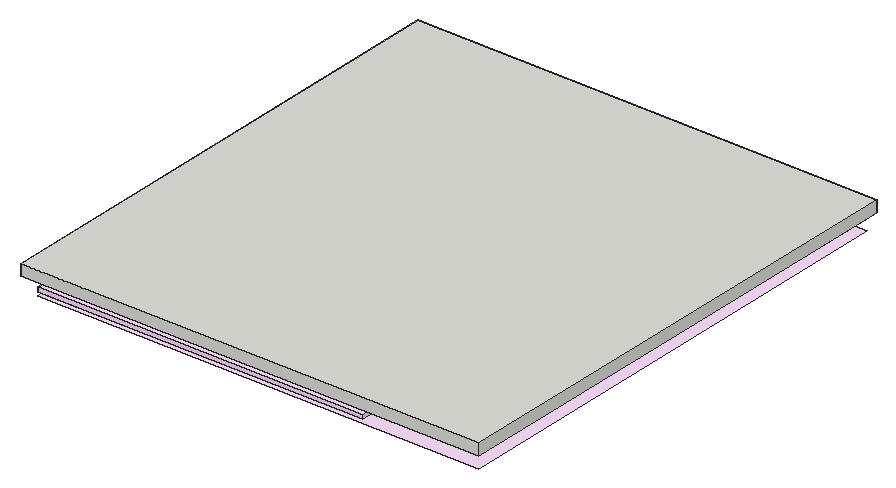
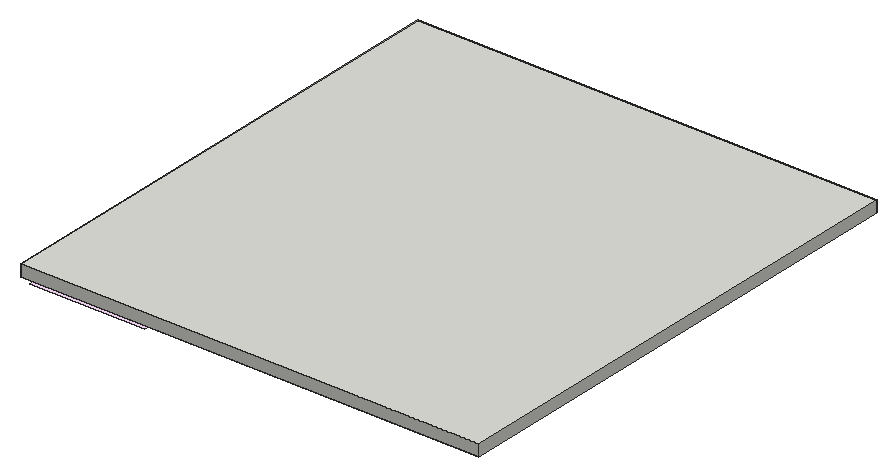
# SketchUp Ruby script. Lengths in inches.
U = 1.inch
M = Sketchup.active_model
def pt(a) = Geom::Point3d.new(a.map { |v| v * U })
def face(e, loops, mat)
  f = e.add_face(loops[0].map { |a| pt(a) })
  loops[1..].each { |l| e.add_face(l.map { |a| pt(a) }).erase! }
  f.material = f.back_material = mat if mat
  f
end
# faces: each face lists its corners as indices into pts; further lists are holes
def faces(e, pts, list, mat = nil) = list.each { |f| face(e, (f[0].is_a?(Array) ? f : [f]).map { |l| l.map { |i| pts[i] } }, mat) }
# xy, xz, yz: faces in a plane at the given z, y or x. An outline is a flat list of corners, or four numbers for a rectangle; further outlines are holes
def ring(l) = l.size == 4 ? [[l[0], l[1]], [l[2], l[1]], [l[2], l[3]], [l[0], l[3]]] : l.each_slice(2).to_a
def flat(e, list, mat, &to3) = list.each { |f| face(e, (f[0].is_a?(Array) ? f : [f]).map { |l| ring(l).map { |u, v| to3.(u, v) } }, mat) }
def xy(e, z, list, mat = nil) = flat(e, list, mat) { |x, y| [x, y, z] }
def xz(e, y, list, mat = nil) = flat(e, list, mat) { |x, z| [x, y, z] }
def yz(e, x, list, mat = nil) = flat(e, list, mat) { |y, z| [x, y, z] }
def lines(e, pts, list) = list.each { |a, b| e.add_line(pt(pts[a]), pt(pts[b])) }
# prism: a flat outline (further loops are holes) pulled along v
def prism(e, loops, v, mat = nil)
  f = face(e, loops, mat); d = Geom::Vector3d.new(v.map { |x| x * U })
  f.pushpull(f.normal.samedirection?(d) ? d.length : -d.length)
end
def box(e, o, s, mat = nil) = prism(e, [[o, [o[0] + s[0], o[1], o[2]], [o[0] + s[0], o[1] + s[1], o[2]], [o[0], o[1] + s[1], o[2]]]], [0, 0, s[2]], mat)
def at(x, y, z, deg = 0) = Geom::Transformation.translation(pt([x, y, z])) * Geom::Transformation.rotation(ORIGIN, Z_AXIS, deg.degrees)
def axes(o, x, y, z) = Geom::Transformation.new([*x, 0, *y, 0, *z, 0, *pt(o).to_a, 1])
def part(name) = M.definitions.add(name)
# library, detail: a bought-in or finely detailed component or shape, given as its bounding box
def library(name, o, s) = part(name).tap { |d| box(d.entities, o, s) }
def detail(e, o, s) = box(e.add_group.entities, o, s)
def put(e, d, t, mat = nil) = e.add_instance(d, t).tap { |i| i.material = mat if mat }
def group(e, t, mat = nil) = e.add_group.tap { |g| g.transformation = t; g.material = mat if mat }.entities
root = M.entities
M.materials.add("[0118_Thistle]").color = [255, 225, 255]
M.materials.add("[Color M00]").color = [255, 255, 255]
xy(root,116.0625,[[[48.73,154.34,48.21,154.4,47.73,154.6,47.32,154.92,47,155.34,46.8,155.82,46.73,156.34,46.8,156.85,47,157.34,47.32,157.75,47.73,158.07,48.21,158.27,48.73,158.34,49.25,158.27,49.73,158.07,50.15,157.75,50.46,157.34,50.66,156.85,50.73,156.34,50.66,155.82,50.46,155.34,50.15,154.92,49.73,154.6,49.25,154.4],[48.73,154.84,49.12,154.89,49.48,155.04,49.79,155.28,50.03,155.59,50.18,155.95,50.23,156.34,50.18,156.72,50.03,157.09,49.79,157.4,49.48,157.64,49.12,157.79,48.73,157.84,48.34,157.79,47.98,157.64,47.67,157.4,47.43,157.09,47.28,156.72,47.23,156.34,47.28,155.95,47.43,155.59,47.67,155.28,47.98,155.04,48.34,154.89]]],"[Color M00]")
xy(root,116.125,[[[32.11,108.44,31.6,108.51,31.11,108.71,30.7,109.03,30.38,109.44,30.18,109.93,30.11,110.44,30.18,110.96,30.38,111.44,30.7,111.86,31.11,112.18,31.6,112.375,32.11,112.44,32.63,112.375,33.11,112.18,33.53,111.86,33.85,111.44,34.05,110.96,34.11,110.44,34.05,109.93,33.85,109.44,33.53,109.03,33.11,108.71,32.63,108.51],[32.11,108.94,32.5,108.99,32.86,109.14,33.17,109.38,33.41,109.69,33.5625,110.06,33.61,110.44,33.5625,110.83,33.41,111.19,33.17,111.5,32.86,111.74,32.5,111.89,32.11,111.94,31.73,111.89,31.36,111.74,31.05,111.5,30.81,111.19,30.66,110.83,30.61,110.44,30.66,110.06,30.81,109.69,31.05,109.38,31.36,109.14,31.73,108.99]],[[178.2,146.39,177.6875,146.46,177.2,146.66,176.79,146.97,176.47,147.39,176.27,147.87,176.2,148.39,176.27,148.91,176.47,149.39,176.79,149.8,177.2,150.12,177.6875,150.32,178.2,150.39,178.72,150.32,179.2,150.12,179.62,149.8,179.9375,149.39,180.14,148.91,180.2,148.39,180.14,147.87,179.9375,147.39,179.62,146.97,179.2,146.66,178.72,146.46],[178.2,146.89,178.59,146.94,178.95,147.09,179.26,147.33,179.5,147.64,179.65,148,179.7,148.39,179.65,148.78,179.5,149.14,179.26,149.45,178.95,149.6875,178.59,149.84,178.2,149.89,177.82,149.84,177.45,149.6875,177.14,149.45,176.91,149.14,176.76,148.78,176.7,148.39,176.76,148,176.91,147.64,177.14,147.33,177.45,147.09,177.82,146.94]],[[126.7,154.34,126.1875,154.4,125.7,154.6,125.29,154.92,124.97,155.34,124.77,155.82,124.7,156.34,124.77,156.85,124.97,157.34,125.29,157.75,125.7,158.07,126.1875,158.27,126.7,158.34,127.22,158.27,127.7,158.07,128.12,157.75,128.44,157.34,128.64,156.85,128.7,156.34,128.64,155.82,128.44,155.34,128.12,154.92,127.7,154.6,127.22,154.4],[126.7,154.82,127.1,154.87,127.46,155.02,127.78,155.26,128.02,155.58,128.17,155.94,128.22,156.34,128.17,156.73,128.02,157.09,127.78,157.41,127.46,157.65,127.1,157.8,126.7,157.85,126.3125,157.8,125.94,157.65,125.63,157.41,125.39,157.09,125.24,156.73,125.1875,156.34,125.24,155.94,125.39,155.58,125.63,155.26,125.94,155.02,126.3125,154.87]]],"[Color M00]")
xy(root,116.1875,[[[160.13,91.36,159.62,91.43,159.13,91.625,158.72,91.94,158.4,92.36,158.2,92.84,158.13,93.36,158.2,93.875,158.4,94.36,158.72,94.77,159.13,95.09,159.62,95.29,160.13,95.36,160.65,95.29,161.13,95.09,161.55,94.77,161.87,94.36,162.07,93.875,162.13,93.36,162.07,92.84,161.87,92.36,161.55,91.94,161.13,91.625,160.65,91.43],[160.13,91.86,160.52,91.91,160.88,92.06,161.19,92.3,161.43,92.61,161.58,92.97,161.63,93.36,161.58,93.75,161.43,94.11,161.19,94.42,160.88,94.66,160.52,94.81,160.13,94.86,159.75,94.81,159.38,94.66,159.07,94.42,158.83,94.11,158.69,93.75,158.63,93.36,158.69,92.97,158.83,92.61,159.07,92.3,159.38,92.06,159.75,91.91]],[[197,180.74,196.49,180.81,196,181,195.59,181.32,195.27,181.74,195.07,182.22,195,182.74,195.07,183.25,195.27,183.74,195.59,184.15,196,184.47,196.49,184.67,197,184.74,197.52,184.67,198,184.47,198.42,184.15,198.74,183.74,198.93,183.25,199,182.74,198.93,182.22,198.74,181.74,198.42,181.32,198,181,197.52,180.81],[197,181.24,197.39,181.29,197.75,181.4375,198.0625,181.68,198.3,181.99,198.45,182.35,198.5,182.74,198.45,183.125,198.3,183.49,198.0625,183.8,197.75,184.04,197.39,184.1875,197,184.24,196.61,184.1875,196.25,184.04,195.94,183.8,195.7,183.49,195.55,183.125,195.5,182.74,195.55,182.35,195.7,181.99,195.94,181.68,196.25,181.4375,196.61,181.29]],[[196.98,236.89,196.46,236.96,195.98,237.17,195.57,237.49,195.26,237.91,195.07,238.39,195,238.91,195.08,239.43,195.28,239.91,195.6,240.32,196.02,240.63,196.51,240.83,197.03,240.89,197.54,240.8125,198.02,240.61,198.43,240.29,198.75,239.87,198.94,239.38,199,238.87,198.93,238.35,198.72,237.87,198.4,237.46,197.98,237.14,197.5,236.95],[196.99,237.39,197.375,237.43,197.74,237.58,198.05,237.82,198.29,238.125,198.45,238.48,198.5,238.87,198.46,239.26,198.3125,239.625,198.08,239.9375,197.77,240.18,197.41,240.33,197.02,240.39,196.63,240.34,196.27,240.2,195.95,239.96,195.71,239.65,195.56,239.29,195.5,238.91,195.55,238.52,195.7,238.15,195.93,237.84,196.24,237.6,196.6,237.44]]],"[Color M00]")
xy(root,116.25,[[178.2,146.89,177.82,146.94,177.45,147.09,177.14,147.33,176.91,147.64,176.76,148,176.7,148.39,176.76,148.78,176.91,149.14,177.14,149.45,177.45,149.6875,177.82,149.84,178.2,149.89,178.59,149.84,178.95,149.6875,179.26,149.45,179.5,149.14,179.65,148.78,179.7,148.39,179.65,148,179.5,147.64,179.26,147.33,178.95,147.09,178.59,146.94]],"[Color M00]")
xy(root,116.3125,[[126.7,154.82,126.3125,154.87,125.94,155.02,125.63,155.26,125.39,155.58,125.24,155.94,125.1875,156.34,125.24,156.73,125.39,157.09,125.63,157.41,125.94,157.65,126.3125,157.8,126.7,157.85,127.1,157.8,127.46,157.65,127.78,157.41,128.02,157.09,128.17,156.73,128.22,156.34,128.17,155.94,128.02,155.58,127.78,155.26,127.46,155.02,127.1,154.87],[48.73,154.84,48.34,154.89,47.98,155.04,47.67,155.28,47.43,155.59,47.28,155.95,47.23,156.34,47.28,156.72,47.43,157.09,47.67,157.4,47.98,157.64,48.34,157.79,48.73,157.84,49.12,157.79,49.48,157.64,49.79,157.4,50.03,157.09,50.18,156.72,50.23,156.34,50.18,155.95,50.03,155.59,49.79,155.28,49.48,155.04,49.12,154.89]],"[Color M00]")
xy(root,116.4375,[[160.13,91.86,159.75,91.91,159.38,92.06,159.07,92.3,158.83,92.61,158.69,92.97,158.63,93.36,158.69,93.75,158.83,94.11,159.07,94.42,159.38,94.66,159.75,94.81,160.13,94.86,160.52,94.81,160.88,94.66,161.19,94.42,161.43,94.11,161.58,93.75,161.63,93.36,161.58,92.97,161.43,92.61,161.19,92.3,160.88,92.06,160.52,91.91],[32.11,108.94,31.73,108.99,31.36,109.14,31.05,109.38,30.81,109.69,30.66,110.06,30.61,110.44,30.66,110.83,30.81,111.19,31.05,111.5,31.36,111.74,31.73,111.89,32.11,111.94,32.5,111.89,32.86,111.74,33.17,111.5,33.41,111.19,33.5625,110.83,33.61,110.44,33.5625,110.06,33.41,109.69,33.17,109.38,32.86,109.14,32.5,108.99]],"[Color M00]")
xy(root,116.5,[[196.99,237.39,196.6,237.44,196.24,237.6,195.93,237.84,195.7,238.15,195.55,238.52,195.5,238.91,195.56,239.29,195.71,239.65,195.95,239.96,196.27,240.2,196.63,240.34,197.02,240.39,197.41,240.33,197.77,240.18,198.08,239.9375,198.3125,239.625,198.46,239.26,198.5,238.87,198.45,238.48,198.29,238.125,198.05,237.82,197.74,237.58,197.375,237.43]],"[Color M00]")
xy(root,116.625,[[197,181.24,196.61,181.29,196.25,181.4375,195.94,181.68,195.7,181.99,195.55,182.35,195.5,182.74,195.55,183.125,195.7,183.49,195.94,183.8,196.25,184.04,196.61,184.1875,197,184.24,197.39,184.1875,197.75,184.04,198.0625,183.8,198.3,183.49,198.45,183.125,198.5,182.74,198.45,182.35,198.3,181.99,198.0625,181.68,197.75,181.4375,197.39,181.29]],"[Color M00]")
xy(root,120,[[[9,0,240,0,240,254.0625,179.62,254.0625,179.62,171,9,171],[51.1875,30.1875,49.62,30.29,48.08,30.6,46.59,31.1,45.1875,31.79,43.88,32.67,42.7,33.7,41.67,34.88,40.79,36.1875,40.1,37.59,39.6,39.08,39.29,40.62,39.1875,42.1875,39.1875,128.8125,39.29,130.38,39.6,131.92,40.1,133.41,40.79,134.8125,41.67,136.12,42.7,137.3,43.88,138.33,45.1875,139.21,46.59,139.9,48.08,140.4,49.62,140.71,51.1875,140.8125,137.43,140.8125,139,140.71,140.54,140.4,142.02,139.9,143.43,139.21,144.74,138.33,145.92,137.3,146.95,136.12,147.82,134.8125,148.52,133.41,149.02,131.92,149.33,130.38,149.43,128.8125,149.43,42.1875,149.33,40.62,149.02,39.08,148.52,37.59,147.82,36.1875,146.95,34.88,145.92,33.7,144.74,32.67,143.43,31.79,142.02,31.1,140.54,30.6,139,30.29,137.43,30.1875]]],"[0118_Thistle]")
p = [[178.2,146.39,116],[177.6875,146.46,116],[177.6875,146.46,116.125],[178.2,146.39,116.125],[178.72,146.46,116],[178.72,146.46,116.125],
  [177.2,146.66,116],[177.2,146.66,116.125],[179.2,146.66,116],[179.2,146.66,116.125],[176.79,146.97,116],[176.79,146.97,116.125],
  [179.62,146.97,116],[179.62,146.97,116.125],[176.47,147.39,116],[176.47,147.39,116.125],[179.9375,147.39,116],[179.9375,147.39,116.125],
  [176.27,147.87,116],[176.27,147.87,116.125],[180.14,147.87,116],[180.14,147.87,116.125],[176.2,148.39,116],[176.2,148.39,116.125],
  [180.2,148.39,116],[180.2,148.39,116.125],[176.27,148.91,116],[176.27,148.91,116.125],[180.14,148.91,116],[180.14,148.91,116.125],
  [176.47,149.39,116],[176.47,149.39,116.125],[179.9375,149.39,116],[179.9375,149.39,116.125],[176.79,149.8,116],[176.79,149.8,116.125],
  [179.62,149.8,116],[179.62,149.8,116.125],[177.2,150.12,116],[177.2,150.12,116.125],[179.2,150.12,116],[179.2,150.12,116.125],
  [177.6875,150.32,116],[177.6875,150.32,116.125],[178.72,150.32,116],[178.72,150.32,116.125],[178.2,150.39,116],[178.2,150.39,116.125],
  [196.98,236.89,116],[196.46,236.96,116],[196.46,236.96,116.1875],[196.98,236.89,116.1875],[197.5,236.95,116],[197.5,236.95,116.1875],
  [195.98,237.17,116],[195.98,237.17,116.1875],[195.57,237.49,116],[195.57,237.49,116.1875],[195.26,237.91,116],[195.26,237.91,116.1875],
  [195.07,238.39,116],[195.07,238.39,116.1875],[195,238.91,116],[195,238.91,116.1875],[195.08,239.43,116],[195.08,239.43,116.1875],
  [32.11,108.94,116.4375],[32.11,108.94,116.125],[31.73,108.99,116.125],[31.73,108.99,116.4375],[32.5,108.99,116.4375],[32.5,108.99,116.125],
  [31.36,109.14,116.125],[31.36,109.14,116.4375],[32.86,109.14,116.4375],[32.86,109.14,116.125],[31.05,109.38,116.125],[31.05,109.38,116.4375],
  [33.17,109.38,116.4375],[33.17,109.38,116.125],[30.81,109.69,116.125],[30.81,109.69,116.4375],[33.41,109.69,116.4375],[33.41,109.69,116.125],
  [30.66,110.06,116.125],[30.66,110.06,116.4375],[33.5625,110.06,116.4375],[33.5625,110.06,116.125],[30.61,110.44,116.125],[30.61,110.44,116.4375],
  [33.61,110.44,116.4375],[33.61,110.44,116.125],[30.66,110.83,116.125],[30.66,110.83,116.4375],[33.5625,110.83,116.4375],[33.5625,110.83,116.125],
  [30.81,111.19,116.125],[30.81,111.19,116.4375],[33.41,111.19,116.4375],[33.41,111.19,116.125],[31.05,111.5,116.125],[31.05,111.5,116.4375],
  [33.17,111.5,116.4375],[33.17,111.5,116.125],[31.36,111.74,116.125],[31.36,111.74,116.4375],[32.86,111.74,116.4375],[32.86,111.74,116.125],
  [31.73,111.89,116.125],[31.73,111.89,116.4375],[32.5,111.89,116.4375],[32.5,111.89,116.125],[32.11,111.94,116.125],[32.11,111.94,116.4375],
  [177.82,146.94,116.25],[177.82,146.94,116.125],[177.45,147.09,116.125],[177.45,147.09,116.25],[178.2,146.89,116.25],[178.2,146.89,116.125],
  [178.59,146.94,116.25],[178.59,146.94,116.125],[178.95,147.09,116.25],[178.95,147.09,116.125],[177.14,147.33,116.125],[177.14,147.33,116.25],
  [179.26,147.33,116.25],[179.26,147.33,116.125],[176.91,147.64,116.125],[176.91,147.64,116.25],[179.5,147.64,116.25],[179.5,147.64,116.125],
  [176.76,148,116.125],[176.76,148,116.25],[179.65,148,116.25],[179.65,148,116.125],[176.7,148.39,116.125],[176.7,148.39,116.25],
  [179.7,148.39,116.25],[179.7,148.39,116.125],[176.76,148.78,116.125],[176.76,148.78,116.25],[179.65,148.78,116.25],[179.65,148.78,116.125],
  [176.91,149.14,116.125],[176.91,149.14,116.25],[179.5,149.14,116.25],[179.5,149.14,116.125],[177.14,149.45,116.125],[177.14,149.45,116.25],
  [179.26,149.45,116.25],[179.26,149.45,116.125],[177.45,149.6875,116.125],[177.45,149.6875,116.25],[178.95,149.6875,116.25],[178.95,149.6875,116.125],
  [177.82,149.84,116.125],[177.82,149.84,116.25],[178.59,149.84,116.25],[178.59,149.84,116.125],[178.2,149.89,116.125],[178.2,149.89,116.25],
  [48.73,154.84,116.3125],[48.73,154.84,116.0625],[48.34,154.89,116.0625],[48.34,154.89,116.3125],[49.12,154.89,116.3125],[49.12,154.89,116.0625],
  [126.7,154.82,116.3125],[126.7,154.82,116.125],[126.3125,154.87,116.125],[126.3125,154.87,116.3125],[127.1,154.87,116.3125],[127.1,154.87,116.125],
  [47.98,155.04,116.0625],[47.98,155.04,116.3125],[49.48,155.04,116.3125],[49.48,155.04,116.0625],[125.94,155.02,116.125],[125.94,155.02,116.3125],
  [127.46,155.02,116.3125],[127.46,155.02,116.125],[47.67,155.28,116.0625],[47.67,155.28,116.3125],[49.79,155.28,116.3125],[49.79,155.28,116.0625],
  [125.63,155.26,116.125],[125.63,155.26,116.3125],[127.78,155.26,116.3125],[127.78,155.26,116.125],[47.43,155.59,116.0625],[47.43,155.59,116.3125],
  [50.03,155.59,116.3125],[50.03,155.59,116.0625],[125.39,155.58,116.125],[125.39,155.58,116.3125],[128.02,155.58,116.3125],[128.02,155.58,116.125],
  [47.28,155.95,116.0625],[47.28,155.95,116.3125],[50.18,155.95,116.3125],[50.18,155.95,116.0625],[125.24,155.94,116.125],[125.24,155.94,116.3125],
  [128.17,155.94,116.3125],[128.17,155.94,116.125],[47.23,156.34,116.0625],[47.23,156.34,116.3125],[50.23,156.34,116.3125],[50.23,156.34,116.0625],
  [125.1875,156.34,116.125],[125.1875,156.34,116.3125],[128.22,156.34,116.3125],[128.22,156.34,116.125],[47.28,156.72,116.0625],[47.28,156.72,116.3125],
  [50.18,156.72,116.3125],[50.18,156.72,116.0625],[125.24,156.73,116.125],[125.24,156.73,116.3125],[128.17,156.73,116.3125],[128.17,156.73,116.125],
  [47.43,157.09,116.0625],[47.43,157.09,116.3125],[50.03,157.09,116.3125],[50.03,157.09,116.0625],[125.39,157.09,116.125],[125.39,157.09,116.3125],
  [128.02,157.09,116.3125],[128.02,157.09,116.125],[47.67,157.4,116.0625],[47.67,157.4,116.3125],[49.79,157.4,116.3125],[49.79,157.4,116.0625],
  [125.63,157.41,116.125],[125.63,157.41,116.3125],[127.78,157.41,116.3125],[127.78,157.41,116.125],[47.98,157.64,116.0625],[47.98,157.64,116.3125],
  [49.48,157.64,116.3125],[49.48,157.64,116.0625],[125.94,157.65,116.125],[125.94,157.65,116.3125],[127.46,157.65,116.3125],[127.46,157.65,116.125],
  [48.34,157.79,116.0625],[48.34,157.79,116.3125],[49.12,157.79,116.3125],[49.12,157.79,116.0625],[126.3125,157.8,116.125],[126.3125,157.8,116.3125],
  [127.1,157.8,116.3125],[127.1,157.8,116.125],[48.73,157.84,116.0625],[48.73,157.84,116.3125],[126.7,157.85,116.125],[126.7,157.85,116.3125],
  [159.75,91.91,116.4375],[159.75,91.91,116.1875],[159.38,92.06,116.1875],[159.38,92.06,116.4375],[160.13,91.86,116.4375],[160.13,91.86,116.1875],
  [160.52,91.91,116.4375],[160.52,91.91,116.1875],[160.88,92.06,116.4375],[160.88,92.06,116.1875],[159.07,92.3,116.1875],[159.07,92.3,116.4375],
  [161.19,92.3,116.4375],[161.19,92.3,116.1875],[158.83,92.61,116.1875],[158.83,92.61,116.4375],[161.43,92.61,116.4375],[161.43,92.61,116.1875],
  [158.69,92.97,116.1875],[158.69,92.97,116.4375],[161.58,92.97,116.4375],[161.58,92.97,116.1875],[158.63,93.36,116.1875],[158.63,93.36,116.4375],
  [161.63,93.36,116.4375],[161.63,93.36,116.1875],[158.69,93.75,116.1875],[158.69,93.75,116.4375],[161.58,93.75,116.4375],[161.58,93.75,116.1875],
  [158.83,94.11,116.1875],[158.83,94.11,116.4375],[161.43,94.11,116.4375],[161.43,94.11,116.1875],[159.07,94.42,116.1875],[159.07,94.42,116.4375],
  [161.19,94.42,116.4375],[161.19,94.42,116.1875],[159.38,94.66,116.1875],[159.38,94.66,116.4375],[160.88,94.66,116.4375],[160.88,94.66,116.1875],
  [159.75,94.81,116.1875],[159.75,94.81,116.4375],[160.52,94.81,116.4375],[160.52,94.81,116.1875],[160.13,94.86,116.1875],[160.13,94.86,116.4375],
  [197,181.24,116.625],[197,181.24,116.1875],[196.61,181.29,116.1875],[196.61,181.29,116.625],[197.39,181.29,116.625],[197.39,181.29,116.1875],
  [196.25,181.4375,116.1875],[196.25,181.4375,116.625],[197.75,181.4375,116.625],[197.75,181.4375,116.1875],[195.94,181.68,116.1875],[195.94,181.68,116.625],
  [198.0625,181.68,116.625],[198.0625,181.68,116.1875],[195.7,181.99,116.1875],[195.7,181.99,116.625],[198.3,181.99,116.625],[198.3,181.99,116.1875],
  [195.55,182.35,116.1875],[195.55,182.35,116.625],[198.45,182.35,116.625],[198.45,182.35,116.1875],[195.5,182.74,116.1875],[195.5,182.74,116.625],
  [198.5,182.74,116.625],[198.5,182.74,116.1875],[195.55,183.125,116.1875],[195.55,183.125,116.625],[198.45,183.125,116.625],[198.45,183.125,116.1875],
  [195.7,183.49,116.1875],[195.7,183.49,116.625],[198.3,183.49,116.625],[198.3,183.49,116.1875],[195.94,183.8,116.1875],[195.94,183.8,116.625],
  [198.0625,183.8,116.625],[198.0625,183.8,116.1875],[196.25,184.04,116.1875],[196.25,184.04,116.625],[197.75,184.04,116.625],[197.75,184.04,116.1875],
  [196.61,184.1875,116.1875],[196.61,184.1875,116.625],[197.39,184.1875,116.625],[197.39,184.1875,116.1875],[197,184.24,116.1875],[197,184.24,116.625],
  [196.6,237.44,116.5],[196.6,237.44,116.1875],[196.24,237.6,116.1875],[196.24,237.6,116.5],[196.99,237.39,116.5],[196.99,237.39,116.1875],
  [197.375,237.43,116.5],[197.375,237.43,116.1875],[197.74,237.58,116.5],[197.74,237.58,116.1875],[195.93,237.84,116.1875],[195.93,237.84,116.5],
  [198.05,237.82,116.5],[198.05,237.82,116.1875],[195.7,238.15,116.1875],[195.7,238.15,116.5],[198.29,238.125,116.5],[198.29,238.125,116.1875],
  [198.45,238.48,116.5],[198.45,238.48,116.1875],[195.55,238.52,116.1875],[195.55,238.52,116.5],[195.5,238.91,116.1875],[195.5,238.91,116.5],
  [198.5,238.87,116.5],[198.5,238.87,116.1875],[195.56,239.29,116.1875],[195.56,239.29,116.5],[198.46,239.26,116.5],[198.46,239.26,116.1875],
  [195.71,239.65,116.1875],[195.71,239.65,116.5],[198.3125,239.625,116.5],[198.3125,239.625,116.1875],[198.08,239.9375,116.5],[198.08,239.9375,116.1875],
  [195.95,239.96,116.1875],[195.95,239.96,116.5],[197.77,240.18,116.5],[197.77,240.18,116.1875],[196.27,240.2,116.1875],[196.27,240.2,116.5],
  [196.63,240.34,116.1875],[196.63,240.34,116.5],[197.41,240.33,116.5],[197.41,240.33,116.1875],[197.02,240.39,116.1875],[197.02,240.39,116.5]]
faces(root,p,[[0,1,2,3],[4,0,3,5],[1,6,7,2],[8,4,5,9],[6,10,11,7],[12,8,9,13],[10,14,15,11],[16,12,13,17],
  [14,18,19,15],[20,16,17,21],[18,22,23,19],[24,20,21,25],[22,26,27,23],[28,24,25,29],[26,30,31,27],[32,28,29,33],
  [30,34,35,31],[36,32,33,37],[34,38,39,35],[40,36,37,41],[38,42,43,39],[44,40,41,45],[42,46,47,43],[46,44,45,47],
  [48,49,50,51],[52,48,51,53],[49,54,55,50],[54,56,57,55],[56,58,59,57],[58,60,61,59],[60,62,63,61],[62,64,65,63],
  [66,67,68,69],[70,71,67,66],[69,68,72,73],[74,75,71,70],[73,72,76,77],[78,79,75,74],[77,76,80,81],[82,83,79,78],
  [81,80,84,85],[86,87,83,82],[85,84,88,89],[90,91,87,86],[89,88,92,93],[94,95,91,90],[93,92,96,97],[98,99,95,94],
  [97,96,100,101],[102,103,99,98],[101,100,104,105],[106,107,103,102],[105,104,108,109],[110,111,107,106],[109,108,112,113],[113,112,111,110],
  [114,115,116,117],[118,119,115,114],[120,121,119,118],[122,123,121,120],[117,116,124,125],[126,127,123,122],[125,124,128,129],[130,131,127,126],
  [129,128,132,133],[134,135,131,130],[133,132,136,137],[138,139,135,134],[137,136,140,141],[142,143,139,138],[141,140,144,145],[146,147,143,142],
  [145,144,148,149],[150,151,147,146],[149,148,152,153],[154,155,151,150],[153,152,156,157],[158,159,155,154],[157,156,160,161],[161,160,159,158],
  [162,163,164,165],[166,167,163,162],[168,169,170,171],[172,173,169,168],[165,164,174,175],[176,177,167,166],[171,170,178,179],[180,181,173,172],
  [175,174,182,183],[184,185,177,176],[179,178,186,187],[188,189,181,180],[183,182,190,191],[192,193,185,184],[187,186,194,195],[196,197,189,188],
  [191,190,198,199],[200,201,193,192],[195,194,202,203],[204,205,197,196],[199,198,206,207],[208,209,201,200],[203,202,210,211],[212,213,205,204],
  [207,206,214,215],[216,217,209,208],[211,210,218,219],[220,221,213,212],[215,214,222,223],[224,225,217,216],[219,218,226,227],[228,229,221,220],
  [223,222,230,231],[232,233,225,224],[227,226,234,235],[236,237,229,228],[231,230,238,239],[240,241,233,232],[235,234,242,243],[244,245,237,236],
  [239,238,246,247],[248,249,241,240],[243,242,250,251],[252,253,245,244],[247,246,254,255],[255,254,249,248],[251,250,256,257],[257,256,253,252],
  [258,259,260,261],[262,263,259,258],[264,265,263,262],[266,267,265,264],[261,260,268,269],[270,271,267,266],[269,268,272,273],[274,275,271,270],
  [273,272,276,277],[278,279,275,274],[277,276,280,281],[282,283,279,278],[281,280,284,285],[286,287,283,282],[285,284,288,289],[290,291,287,286],
  [289,288,292,293],[294,295,291,290],[293,292,296,297],[298,299,295,294],[297,296,300,301],[302,303,299,298],[301,300,304,305],[305,304,303,302],
  [306,307,308,309],[310,311,307,306],[309,308,312,313],[314,315,311,310],[313,312,316,317],[318,319,315,314],[317,316,320,321],[322,323,319,318],
  [321,320,324,325],[326,327,323,322],[325,324,328,329],[330,331,327,326],[329,328,332,333],[334,335,331,330],[333,332,336,337],[338,339,335,334],
  [337,336,340,341],[342,343,339,338],[341,340,344,345],[346,347,343,342],[345,344,348,349],[350,351,347,346],[349,348,352,353],[353,352,351,350],
  [354,355,356,357],[358,359,355,354],[360,361,359,358],[362,363,361,360],[357,356,364,365],[366,367,363,362],[365,364,368,369],[370,371,367,366],
  [372,373,371,370],[369,368,374,375],[375,374,376,377],[378,379,373,372],[377,376,380,381],[382,383,379,378],[381,380,384,385],[386,387,383,382],
  [388,389,387,386],[385,384,390,391],[392,393,389,388],[391,390,394,395],[395,394,396,397],[398,399,393,392],[397,396,400,401],[401,400,399,398]],"[Color M00]")
g1 = group(root,at(9,0,122),"[0118_Thistle]")
box(g1,[0,0,0],[170.45,171,2])
g2 = group(root,at(0,0,126))
box(g2,[0,0,0],[240,260.0625,6])
